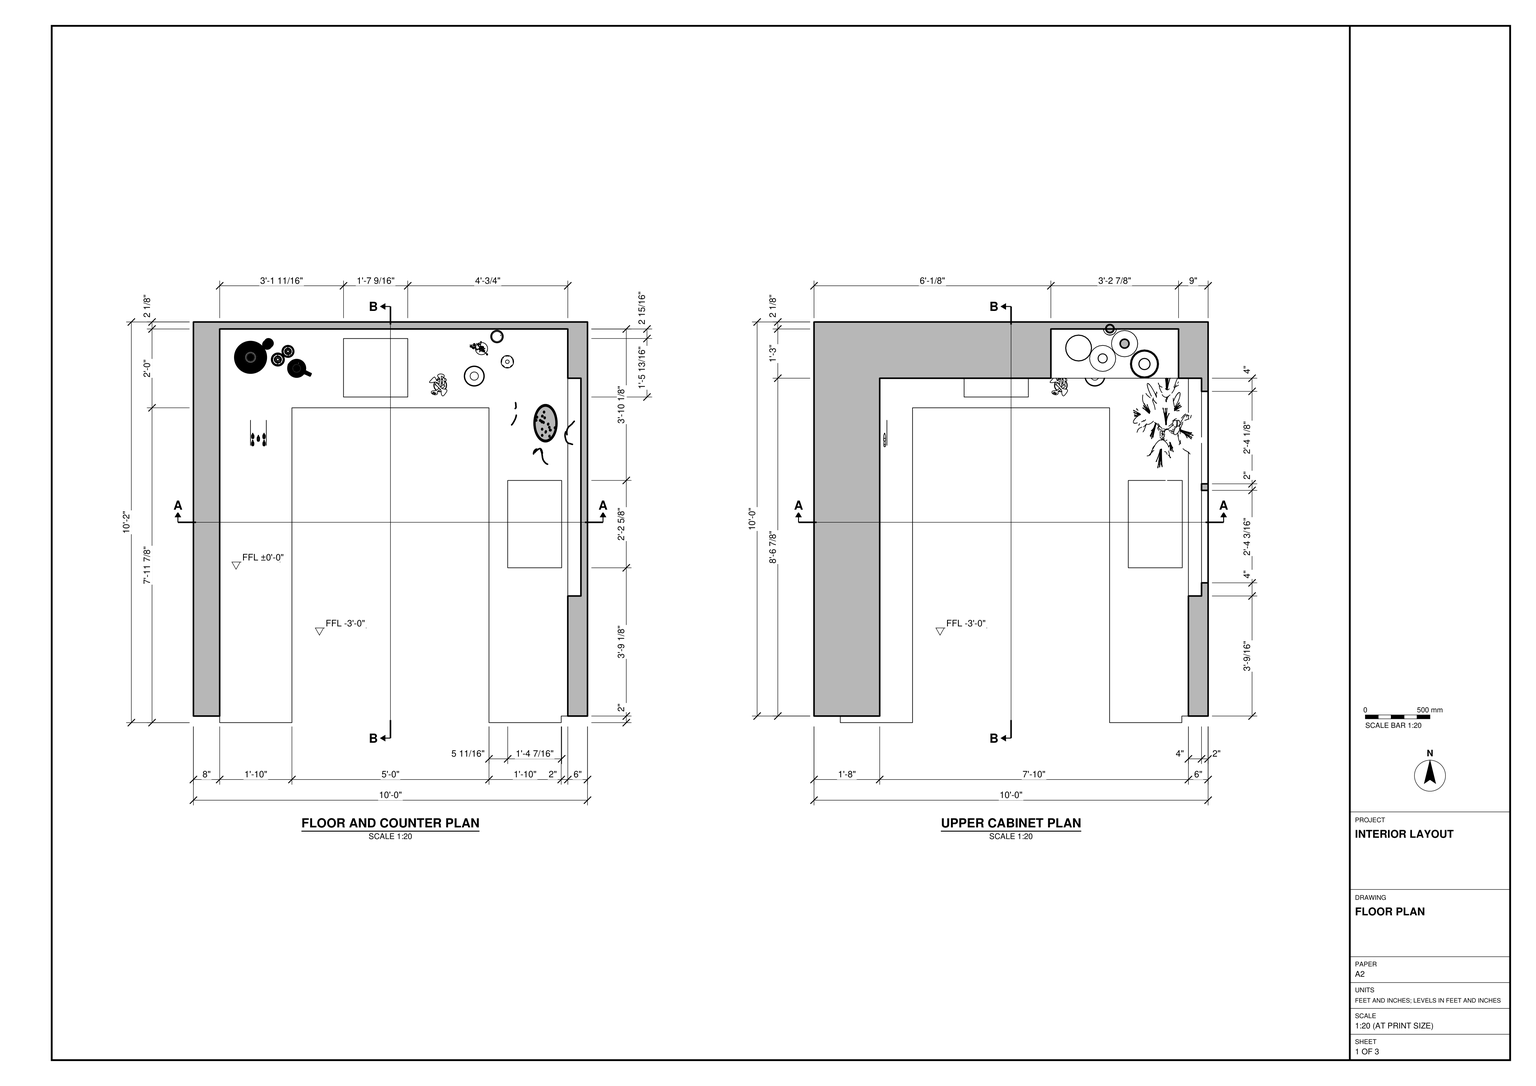
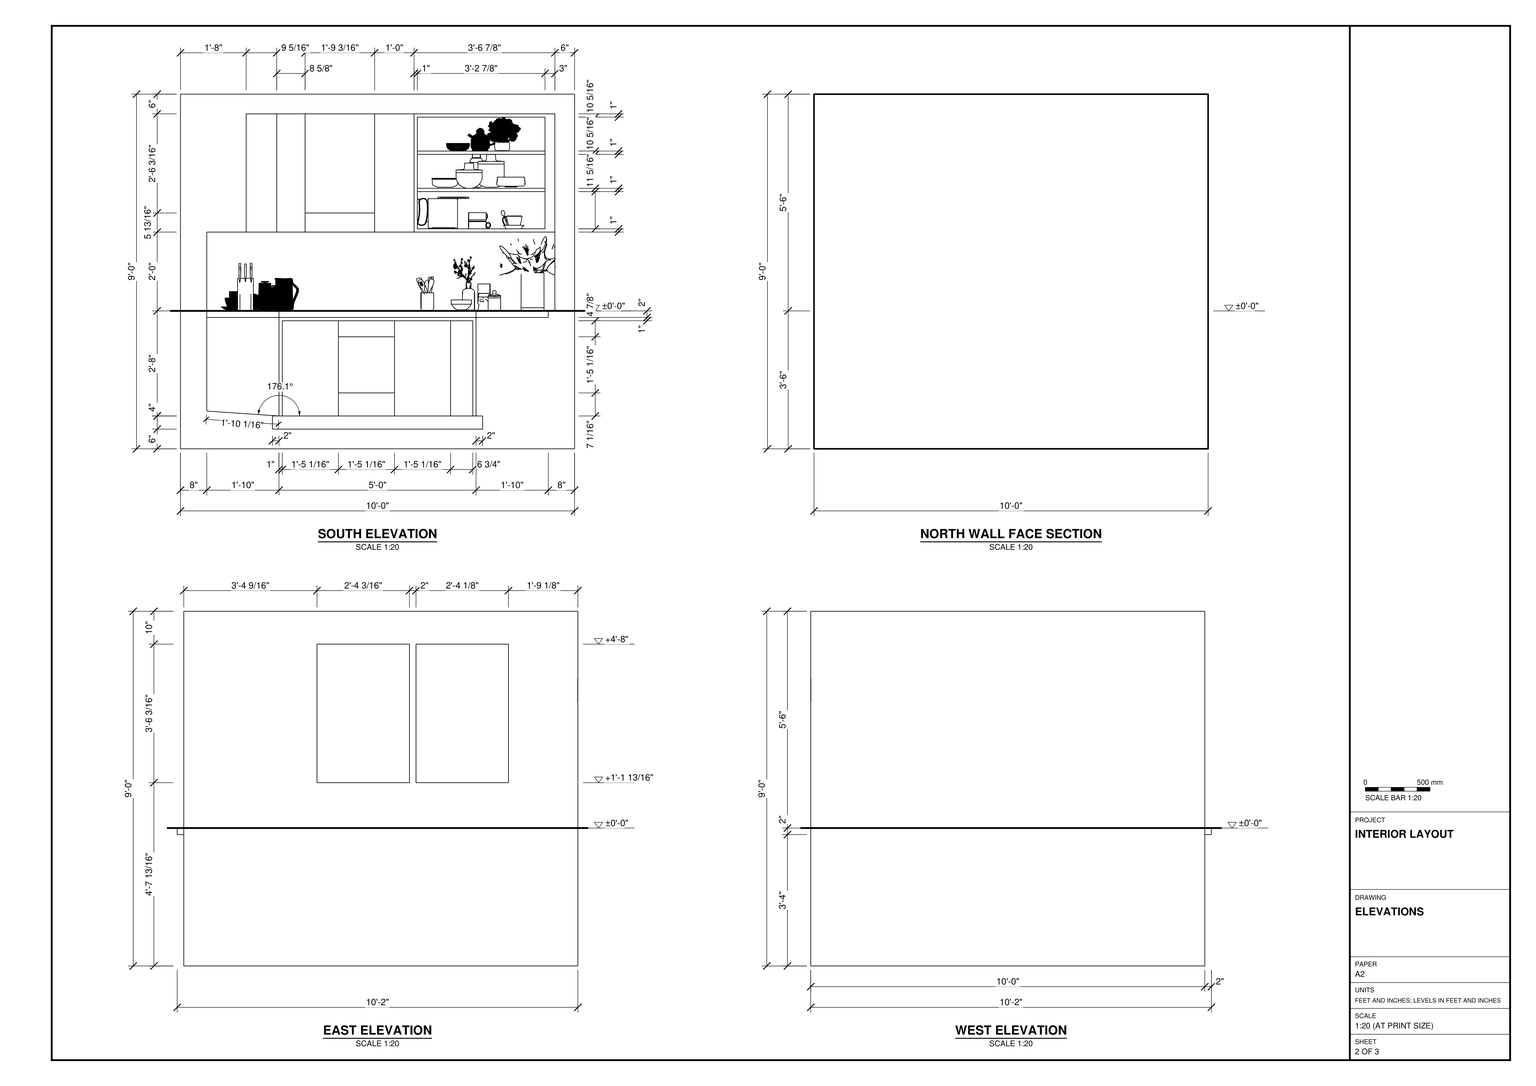
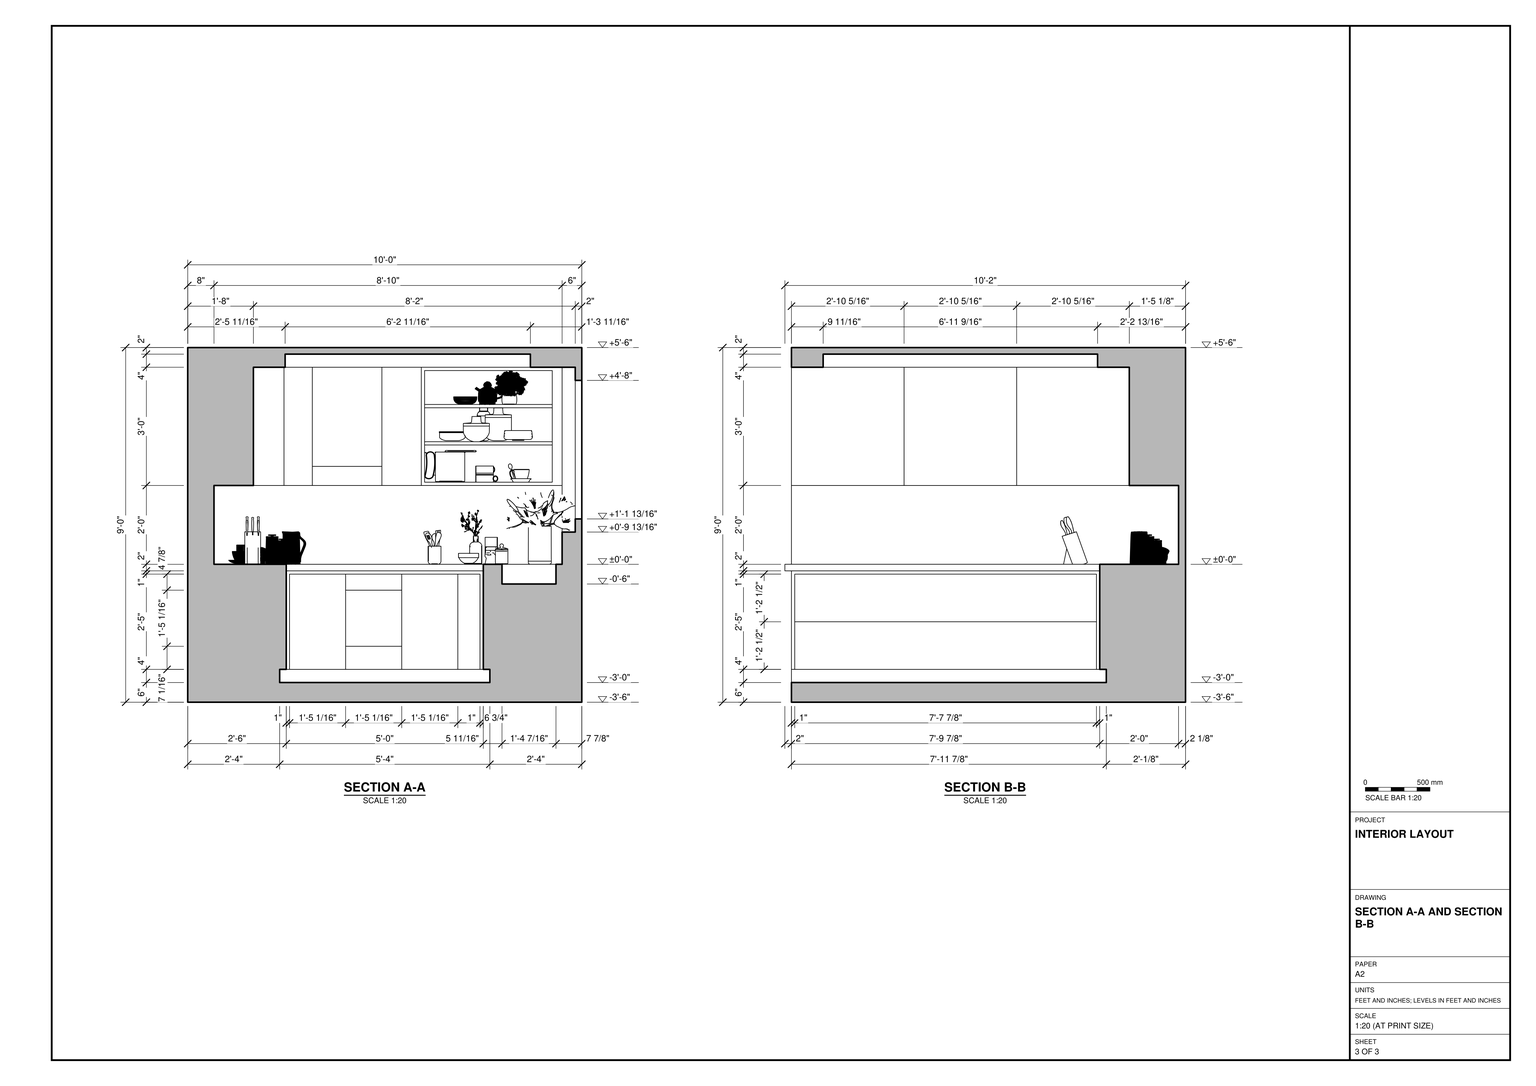
Build the kitchen interior in SketchUp from task_files/diagram_01.pdf. Work in feet and inches. The overall dimensions are 10'-0" along X, 10'-2" along Y and 9'-0" high. Use the single level ±0'-0" as the drawing datum: the counter surface aligns with this level, and the aisle floor is at -3'-0".

Leave the south end open. Model the floor, overhead slab and enclosing walls with the thicknesses and profiles shown in plan and section. Form the paired openings in the east wall above the counter. Run the base cabinets and worktop along both sides and across the back, leaving the central aisle clear. Include the east counter basin, the rectangular feature on the back worktop, the cabinet doors, drawer fronts and plinths. Fit upper cabinets along the west and north walls, with the open shelving at the east end of the north run. Follow the elevations for the cabinet divisions and the sections for the clearance above the counter.

Decor and loose items on the counters and shelves may be any suitable library components. Keep shell elements and each joinery piece in separate groups or components, and use components for repeated parts. Save one SketchUp model as output_files/u_shaped_kitchen_with_fitted_cabinets_and_open_shelving.skp.

# SketchUp Ruby script. Lengths in inches.
U = 1.inch
M = Sketchup.active_model
def pt(a) = Geom::Point3d.new(a.map { |v| v * U })
def face(e, loops, mat)
  f = e.add_face(loops[0].map { |a| pt(a) })
  loops[1..].each { |l| e.add_face(l.map { |a| pt(a) }).erase! }
  f.material = f.back_material = mat if mat
  f
end
# faces: each face lists its corners as indices into pts; further lists are holes
def faces(e, pts, list, mat = nil) = list.each { |f| face(e, (f[0].is_a?(Array) ? f : [f]).map { |l| l.map { |i| pts[i] } }, mat) }
# xy, xz, yz: faces in a plane at the given z, y or x. An outline is a flat list of corners, or four numbers for a rectangle; further outlines are holes
def ring(l) = l.size == 4 ? [[l[0], l[1]], [l[2], l[1]], [l[2], l[3]], [l[0], l[3]]] : l.each_slice(2).to_a
def flat(e, list, mat, &to3) = list.each { |f| face(e, (f[0].is_a?(Array) ? f : [f]).map { |l| ring(l).map { |u, v| to3.(u, v) } }, mat) }
def xy(e, z, list, mat = nil) = flat(e, list, mat) { |x, y| [x, y, z] }
def xz(e, y, list, mat = nil) = flat(e, list, mat) { |x, z| [x, y, z] }
def yz(e, x, list, mat = nil) = flat(e, list, mat) { |y, z| [x, y, z] }
def lines(e, pts, list) = list.each { |a, b| e.add_line(pt(pts[a]), pt(pts[b])) }
# prism: a flat outline (further loops are holes) pulled along v
def prism(e, loops, v, mat = nil)
  f = face(e, loops, mat); d = Geom::Vector3d.new(v.map { |x| x * U })
  f.pushpull(f.normal.samedirection?(d) ? d.length : -d.length)
end
def box(e, o, s, mat = nil) = prism(e, [[o, [o[0] + s[0], o[1], o[2]], [o[0] + s[0], o[1] + s[1], o[2]], [o[0], o[1] + s[1], o[2]]]], [0, 0, s[2]], mat)
def at(x, y, z, deg = 0) = Geom::Transformation.translation(pt([x, y, z])) * Geom::Transformation.rotation(ORIGIN, Z_AXIS, deg.degrees)
def axes(o, x, y, z) = Geom::Transformation.new([*x, 0, *y, 0, *z, 0, *pt(o).to_a, 1])
def part(name) = M.definitions.add(name)
# library, detail: a bought-in or finely detailed component or shape, given as its bounding box
def library(name, o, s) = part(name).tap { |d| box(d.entities, o, s) }
def detail(e, o, s) = box(e.add_group.entities, o, s)
def put(e, d, t, mat = nil) = e.add_instance(d, t).tap { |i| i.material = mat if mat }
def group(e, t, mat = nil) = e.add_group.tap { |g| g.transformation = t; g.material = mat if mat }.entities
root = M.entities
M.materials.add("[0035_Tan]").color = [209, 179, 140]
M.materials.add("[0038_Orange]1").color = [255, 165, 0]
M.materials.add("[0046_Gold]").color = [255, 214, 0]
M.materials.add("[0053_Ivory]").color = [255, 255, 240]
M.materials.add("[0137_Black]").color = [0, 0, 0]
M.materials.add("[Translucent Glass Gray]").color = [128, 128, 128]
M.materials["[Translucent Glass Gray]"].alpha = 0.5
M.materials.add("[Wood Veneer 01]").color = [84, 49, 25]
M.materials.add("[Wood Veneer 01]1").color = [63, 37, 19]
M.materials.add("[Wood Veneer 01]2").color = [120, 70, 37]
c1 = library("Untitled (2)",[-0.59,0,0],[15.67,17.07,16.5])
c2 = library("Florero (1)",[0,-9.1,0],[22.375,11.9,13.13])
c3 = library("Drinkware set",[-0.57,0,0],[14.27,24.52,9.91])
c4 = library("UTENCILIOS",[-3.38,-3.35,0],[5.31,6.7,10.38])
c5 = library("Grupo3\#1",[-2.41,-4.18,0],[4.82,8.16,14.49])
c6 = library("KITCHEN+ITEMS+(30)",[-0.14,0,0],[4.76,4.15,3.43])
c7 = library("Shelf decor arrangement",[-1.72,1.64,0],[13.78,24.1,11.69])
c8 = library("bowls",[-0.39,1.3,-1.14],[28.37,17.08,12.97])
c9 = library("Cups",[28.29,22.05,0],[8.59,8.59,5.51])
c10 = library("Group\#37",[0,0,0],[361.72,361.72,19.96])
c11 = library("Group\#34",[0,0,0],[349.75,349.75,408.25])
c12 = library("Group\#35",[0,0,0],[125.85,31.61,370.5])
c13 = part("cup")
g1 = group(c13.entities,at(-289.39,-196.58,0))
put(g1,c10,axes([237.34,0,430.07],[1,0,0],[0,1,0],[0,0,-1]))
g2 = group(g1,at(0,8.64,0),"[0038_Orange]1")
put(g2,c11,at(120.92,0,0),"[0046_Gold]")
put(g2,c12,at(0,159.1875,44.14),"[0035_Tan]")
xy(root,0,[[0,2,120,122]])
xy(root,6,[[28,2,92,97.875]],"[0053_Ivory]")
xy(root,10,[[28,2,30,97.875],[90,2,92,95.875],[30,95.875,92,97.875]])
xy(root,36,[[95.7,47.15,112.14,73.75]],"[Wood Veneer 01]2")
xy(root,40,[[8,0,30,2],[90,0,112,2]])
xy(root,42,[[[8,0,30,0,30,95.875,90,95.875,90,0,112,0,112,2,114,2,114,119.875,8,119.875],[95.7,47.15,112.14,73.75],[45.7,99.15,65.26,116.96]]],"[0053_Ivory]")
xy(root,42,[[45.7,99.15,65.26,116.96]],"[0137_Black]")
xy(root,51.8125,[[114,38.5625,118,104.875]],"[0053_Ivory]")
xy(root,55.8125,[[118,42.5625,120,70.72],[118,72.72,120,100.875]],"[Wood Veneer 01]1")
xy(root,66,[[8,2,8,119.875,23,119.875,23,104.875,20,104.875,20,2],[23,104.875,114,119.875]],"[0053_Ivory]")
xy(root,67,[[72.125,104.875,111,119.875]],"[Wood Veneer 01]1")
xy(root,78.33,[[72.125,104.875,74.125,119.875],[74.125,104.875,111,119.875]],"[Wood Veneer 01]")
xy(root,79.33,[[72.125,104.875,111,119.875]],"[Wood Veneer 01]1")
xy(root,89.67,[[72.125,104.875,74.125,119.875],[74.125,104.875,111,119.875]],"[Wood Veneer 01]")
xy(root,90.67,[[72.125,104.875,111,119.875]],"[Wood Veneer 01]")
xy(root,98,[[118,42.5625,120,70.72],[118,72.72,120,100.875]],"[Wood Veneer 01]1")
xy(root,101,[[72.125,104.875,74.125,119.875],[74.125,104.875,111,119.875]],"[Wood Veneer 01]")
xy(root,102,[[[20,2,114,104.875],[29.66,11.66,104.34,95.22]],[114,38.5625,118,104.875]],"[0053_Ivory]")
xy(root,106,[[29.66,11.66,104.34,95.22]],"[0053_Ivory]")
xy(root,108,[[0,2,120,122]],"[0053_Ivory]")
xz(root,0,[[8,40,30,42],[90,40,112,42]],"[0053_Ivory]")
xz(root,2,[[[0,0,120,108],[28,6,28,10,30,10,8,11.5,8,66,20,66,20,102,114,102,114,42,112,42,112,40,90,40,90,10,92,10,92,6]]],"[0053_Ivory]")
xz(root,2,[[30,10,30,40,8,40,8,11.5]],"[Wood Veneer 01]2")
xz(root,11.66,[[29.66,102,104.34,106]],"[0053_Ivory]")
xz(root,38.5625,[[114,51.8125,118,102]],"[0053_Ivory]")
xz(root,42.5625,[[118,55.8125,120,98]],"[Wood Veneer 01]1")
xz(root,47.15,[[95.7,36,112.14,42]],"[Wood Veneer 01]2")
xz(root,70.72,[[118,55.8125,120,98]],"[Wood Veneer 01]1")
xz(root,72.72,[[118,55.8125,120,98]],"[Wood Veneer 01]1")
xz(root,73.75,[[95.7,36,112.14,42]],"[Wood Veneer 01]2")
xz(root,95.22,[[29.66,102,104.34,106]],"[0053_Ivory]")
xz(root,95.875,[[30,40,90,42]])
xz(root,95.875,[[48.08,17.03,65.17,34.11]],"[Translucent Glass Gray]")
xz(root,95.875,[[30,10,31,10,31,39,89,39,89,10,90,10,90,40,30,40],[31,10,48.08,39],[48.08,10,65.17,17.03],[65.17,10,82.25,39],[82.25,10,89,39],
  [48.08,34.11,65.17,39]],"[Wood Veneer 01]")
xz(root,97.875,[[28,6,92,10]],"[0053_Ivory]")
xz(root,100.875,[[118,55.8125,120,98]],"[Wood Veneer 01]1")
xz(root,104.875,[[114,51.8125,118,102],[20,66,29.3125,102],[29.3125,66,37.9375,102],[59.125,66,71.125,102],[37.9375,71.82,59.125,102]],"[0053_Ivory]")
xz(root,104.875,[[37.9375,66,59.125,71.82]],"[0137_Black]")
xz(root,104.875,[[[71.125,66,114,102],[72.125,67,111,101]],[72.125,78.33,111,79.33],[72.125,89.67,111,90.67]],"[Wood Veneer 01]")
xz(root,119.875,[[8,42,114,66]],"[0053_Ivory]")
xz(root,119.875,[[72.125,67,111,78.33],[72.125,79.33,111,89.67],[72.125,90.67,111,101]],"[Wood Veneer 01]")
xz(root,122,[[0,0,120,108]],"[0053_Ivory]")
yz(root,0,[[2,0,122,108]],"[0053_Ivory]")
yz(root,8,[[0,40,2,42]])
yz(root,8,[[2,42,119.875,66]],"[0053_Ivory]")
yz(root,20,[[2,66,36.29,102],[36.29,66,70.58,102],[70.58,66,104.875,102]],"[0053_Ivory]")
yz(root,28,[[2,6,97.875,10]],"[0053_Ivory]")
yz(root,29.66,[[11.66,102,95.22,106]],"[0053_Ivory]")
yz(root,30,[[0,40,95.875,42]],"[0053_Ivory]")
yz(root,30,[[2,10,3,10,3,39,94.875,39,94.875,10,95.875,10,95.875,40,2,40],[3,10,94.875,24.5],[3,24.5,94.875,39]],"[Wood Veneer 01]")
yz(root,72.125,[[104.875,67,119.875,78.33],[104.875,79.33,119.875,89.67],[104.875,90.67,119.875,101]],"[Wood Veneer 01]")
yz(root,90,[[0,40,95.875,42]],"[0053_Ivory]")
yz(root,90,[[2,10,2,40,95.875,40,95.875,10,94.875,10,94.875,39,3,39,3,10],[3,10,21.375,39],[21.375,10,39.75,39],[39.75,10,58.125,39],[58.125,10,76.5,39],
  [76.5,10,94.875,39]],"[Wood Veneer 01]")
yz(root,92,[[2,6,97.875,10]],"[0053_Ivory]")
yz(root,95.7,[[47.15,36,73.75,42]],"[Wood Veneer 01]2")
yz(root,104.34,[[11.66,102,95.22,106]],"[0053_Ivory]")
yz(root,111,[[104.875,67,119.875,78.33],[104.875,79.33,119.875,89.67],[104.875,90.67,119.875,101]],"[Wood Veneer 01]")
yz(root,112,[[0,40,2,42]])
yz(root,112.14,[[47.15,36,73.75,42]],"[Wood Veneer 01]2")
yz(root,114,[[2,42,2,102,38.5625,102,38.5625,51.8125,104.875,51.8125,104.875,66,119.875,66,119.875,42]],"[0053_Ivory]")
yz(root,118,[[[38.5625,51.8125,104.875,102],[42.5625,55.8125,100.875,98]],[70.72,55.8125,72.72,98]],"[Wood Veneer 01]1")
yz(root,120,[[[2,0,122,108],[42.5625,55.8125,70.72,98],[72.72,55.8125,100.875,98]]],"[0053_Ivory]")
yz(root,120,[[42.5625,55.8125,70.72,98],[72.72,55.8125,100.875,98]],"[Translucent Glass Gray]")
put(root,c1,at(82.43,102.44,42))
put(root,c2,axes([73.22,102.83,42],[2.05209,0,0],[0,3.3312,0],[0,0,1.78598]))
put(root,c3,at(12.47,117.02,42,-90))
put(root,c4,at(75.28,102.83,42))
put(root,c5,at(19.79,88.13,42))
put(root,c6,axes([97.65,105.98,67],[1.5,0,0],[0,1.86,0],[0,0,1.69]))
put(root,c7,axes([79.33,116.94,90.67],[0,-1,0],[1,0,0],[0,0,0.88394]))
put(root,c8,at(76.97,103.57,80.47))
put(root,c9,at(58.28,87.76,66.41))
put(root,c13,axes([79.72,114.21,67],[0.02625,0,0],[0,0.03708,0],[0,0,0.02248]))
